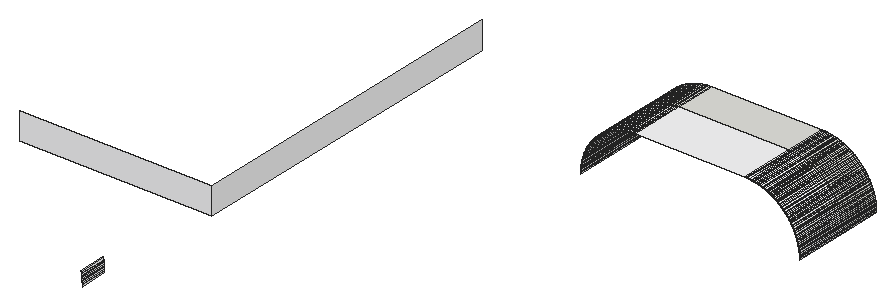
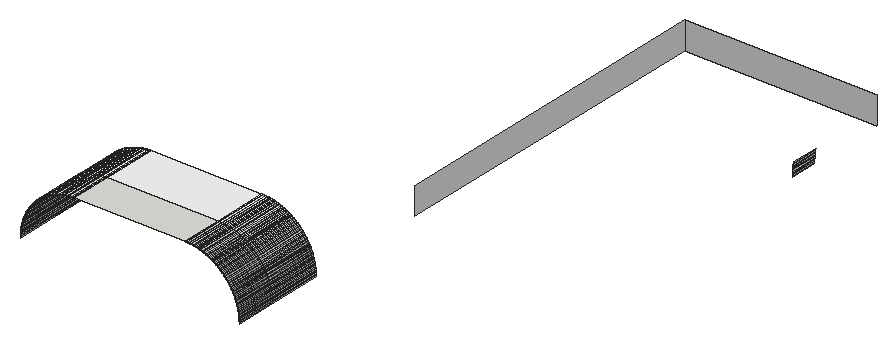
# SketchUp Ruby script. Lengths in inches.
U = 1.inch
M = Sketchup.active_model
def pt(a) = Geom::Point3d.new(a.map { |v| v * U })
def face(e, loops, mat)
  f = e.add_face(loops[0].map { |a| pt(a) })
  loops[1..].each { |l| e.add_face(l.map { |a| pt(a) }).erase! }
  f.material = f.back_material = mat if mat
  f
end
# faces: each face lists its corners as indices into pts; further lists are holes
def faces(e, pts, list, mat = nil) = list.each { |f| face(e, (f[0].is_a?(Array) ? f : [f]).map { |l| l.map { |i| pts[i] } }, mat) }
# xy, xz, yz: faces in a plane at the given z, y or x. An outline is a flat list of corners, or four numbers for a rectangle; further outlines are holes
def ring(l) = l.size == 4 ? [[l[0], l[1]], [l[2], l[1]], [l[2], l[3]], [l[0], l[3]]] : l.each_slice(2).to_a
def flat(e, list, mat, &to3) = list.each { |f| face(e, (f[0].is_a?(Array) ? f : [f]).map { |l| ring(l).map { |u, v| to3.(u, v) } }, mat) }
def xy(e, z, list, mat = nil) = flat(e, list, mat) { |x, y| [x, y, z] }
def xz(e, y, list, mat = nil) = flat(e, list, mat) { |x, z| [x, y, z] }
def yz(e, x, list, mat = nil) = flat(e, list, mat) { |y, z| [x, y, z] }
def lines(e, pts, list) = list.each { |a, b| e.add_line(pt(pts[a]), pt(pts[b])) }
# prism: a flat outline (further loops are holes) pulled along v
def prism(e, loops, v, mat = nil)
  f = face(e, loops, mat); d = Geom::Vector3d.new(v.map { |x| x * U })
  f.pushpull(f.normal.samedirection?(d) ? d.length : -d.length)
end
def box(e, o, s, mat = nil) = prism(e, [[o, [o[0] + s[0], o[1], o[2]], [o[0] + s[0], o[1] + s[1], o[2]], [o[0], o[1] + s[1], o[2]]]], [0, 0, s[2]], mat)
def at(x, y, z, deg = 0) = Geom::Transformation.translation(pt([x, y, z])) * Geom::Transformation.rotation(ORIGIN, Z_AXIS, deg.degrees)
def axes(o, x, y, z) = Geom::Transformation.new([*x, 0, *y, 0, *z, 0, *pt(o).to_a, 1])
def part(name) = M.definitions.add(name)
# library, detail: a bought-in or finely detailed component or shape, given as its bounding box
def library(name, o, s) = part(name).tap { |d| box(d.entities, o, s) }
def detail(e, o, s) = box(e.add_group.entities, o, s)
def put(e, d, t, mat = nil) = e.add_instance(d, t).tap { |i| i.material = mat if mat }
def group(e, t, mat = nil) = e.add_group.tap { |g| g.transformation = t; g.material = mat if mat }.entities
root = M.entities
M.materials.add("[Quartz Light Grey]").color = [251, 251, 252]
xy(root,222,[[245.6875,283,245.84,292],[245.84,283,246,292],[246,283,270,292],[270,283,270.16,292],[270.16,283,270.3125,292]])
xy(root,222,[[245.6875,271,245.84,283],[245.84,271,246,283],[246,271,270,283],[270,271,270.16,283],[270.16,271,270.3125,283]],"[Quartz Light Grey]")
xz(root,195,[[172,228,214,234]],"[Quartz Light Grey]")
yz(root,191.99,[[187,210.47,193,210.71]],"[Quartz Light Grey]")
yz(root,192,[[187,210,193,210.24]],"[Quartz Light Grey]")
yz(root,214,[[195,228,269,234]],"[Quartz Light Grey]")
yz(root,234,[[283,210,292,210.16],[283,210.16,292,210.3125]])
yz(root,234,[[271,210,283,210.16],[271,210.16,283,210.3125]],"[Quartz Light Grey]")
yz(root,282,[[283,210,292,210.16],[283,210.16,292,210.3125]])
yz(root,282,[[271,210,283,210.16],[271,210.16,283,210.3125]],"[Quartz Light Grey]")
p = [[191.99,187,210.47],[191.99,193,210.47],[192,193,210.24],[192,187,210.24],[234,283,210.3125],[234.01,283,210.47],
  [234.01,271,210.47],[234,271,210.3125],[281.99,283,210.47],[282,283,210.3125],[282,271,210.3125],[281.99,271,210.47],
  [234.01,292,210.47],[234.01,283,210.47],[234,283,210.3125],[234,292,210.3125],[282,292,210.3125],[282,283,210.3125],
  [281.99,283,210.47],[281.99,292,210.47],[234.02,283,210.63],[234.02,271,210.63],[281.98,283,210.63],[281.98,271,210.63],
  [234.02,292,210.63],[234.02,283,210.63],[281.98,283,210.63],[281.98,292,210.63],[234.03,283,210.78],[234.03,271,210.78],
  [281.97,283,210.78],[281.97,271,210.78],[234.03,292,210.78],[234.03,283,210.78],[281.97,283,210.78],[281.97,292,210.78],
  [191.98,187,210.94],[191.98,193,210.94],[191.99,193,210.71],[191.99,187,210.71],[234.04,283,210.94],[234.04,271,210.94],
  [281.96,283,210.94],[281.96,271,210.94],[234.04,292,210.94],[234.04,283,210.94],[281.96,283,210.94],[281.96,292,210.94],
  [191.96,187,211.18],[191.96,193,211.18],[234.05,283,211.1],[234.05,271,211.1],[281.95,283,211.1],[281.95,271,211.1],
  [234.05,292,211.1],[234.05,283,211.1],[281.95,283,211.1],[281.95,292,211.1],[234.07,283,211.25],[234.07,271,211.25],
  [281.93,283,211.25],[281.93,271,211.25],[234.07,292,211.25],[234.07,283,211.25],[281.93,283,211.25],[281.93,292,211.25],
  [191.94,187,211.41],[191.94,193,211.41],[234.08,283,211.41],[234.08,271,211.41],[281.92,283,211.41],[281.92,271,211.41],
  [234.08,292,211.41],[234.08,283,211.41],[281.92,283,211.41],[281.92,292,211.41],[191.92,187,211.65],[191.92,193,211.65],
  [234.1,283,211.57],[234.1,271,211.57],[281.9,283,211.57],[281.9,271,211.57],[234.1,292,211.57],[234.1,283,211.57],
  [281.9,283,211.57],[281.9,292,211.57],[191.9,187,211.88],[191.9,193,211.88],[234.125,283,211.72],[234.125,271,211.72],
  [281.875,283,211.72],[281.875,271,211.72],[234.125,292,211.72],[234.125,283,211.72],[281.875,283,211.72],[281.875,292,211.72],
  [234.15,283,211.88],[234.15,271,211.88],[281.85,283,211.88],[281.85,271,211.88],[234.15,292,211.88],[234.15,283,211.88],
  [281.85,283,211.88],[281.85,292,211.88],[191.875,187,212.12],[191.875,193,212.12],[234.17,283,212.03],[234.17,271,212.03],
  [281.83,283,212.03],[281.83,271,212.03],[234.17,292,212.03],[234.17,283,212.03],[281.83,283,212.03],[281.83,292,212.03],
  [234.2,283,212.1875],[234.2,271,212.1875],[281.8,283,212.1875],[281.8,271,212.1875],[234.2,292,212.1875],[234.2,283,212.1875],
  [281.8,283,212.1875],[281.8,292,212.1875],[191.85,187,212.35],[191.85,193,212.35],[234.23,283,212.34],[234.23,271,212.34],
  [281.77,283,212.34],[281.77,271,212.34],[234.23,292,212.34],[234.23,283,212.34],[281.77,283,212.34],[281.77,292,212.34],
  [191.8125,187,212.58],[191.8125,193,212.58],[234.26,283,212.49],[234.26,271,212.49],[281.74,283,212.49],[281.74,271,212.49],
  [234.26,292,212.49],[234.26,283,212.49],[281.74,283,212.49],[281.74,292,212.49],[234.3,283,212.65],[234.3,271,212.65],
  [281.7,283,212.65],[281.7,271,212.65],[234.3,292,212.65],[234.3,283,212.65],[281.7,283,212.65],[281.7,292,212.65],
  [191.78,187,212.82],[191.78,193,212.82],[234.33,283,212.8],[234.33,271,212.8],[281.67,283,212.8],[281.67,271,212.8],
  [234.33,292,212.8],[234.33,283,212.8],[281.67,283,212.8],[281.67,292,212.8],[191.74,187,213.05],[191.74,193,213.05],
  [234.37,283,212.95],[234.37,271,212.95],[281.63,283,212.95],[281.63,271,212.95],[234.37,292,212.95],[234.37,283,212.95],
  [281.63,283,212.95],[281.63,292,212.95],[234.41,283,213.11],[234.41,271,213.11],[281.59,283,213.11],[281.59,271,213.11],
  [234.41,292,213.11],[234.41,283,213.11],[281.59,283,213.11],[281.59,292,213.11],[234.45,283,213.26],[234.45,271,213.26],
  [281.55,283,213.26],[281.55,271,213.26],[234.45,292,213.26],[234.45,283,213.26],[281.55,283,213.26],[281.55,292,213.26],
  [234.49,283,213.41],[234.49,271,213.41],[281.51,283,213.41],[281.51,271,213.41],[234.49,292,213.41],[234.49,283,213.41],
  [281.51,283,213.41],[281.51,292,213.41],[234.54,283,213.56],[234.54,271,213.56],[281.46,283,213.56],[281.46,271,213.56],
  [234.54,292,213.56],[234.54,283,213.56],[281.46,283,213.56],[281.46,292,213.56],[234.59,283,213.71],[234.59,271,213.71],
  [281.41,283,213.71],[281.41,271,213.71],[234.59,292,213.71],[234.59,283,213.71],[281.41,283,213.71],[281.41,292,213.71],
  [234.64,283,213.86],[234.64,271,213.86],[281.36,283,213.86],[281.36,271,213.86],[234.64,292,213.86],[234.64,283,213.86],
  [281.36,283,213.86],[281.36,292,213.86],[234.6875,283,214.01],[234.6875,271,214.01],[281.3125,283,214.01],[281.3125,271,214.01],
  [234.6875,292,214.01],[234.6875,283,214.01],[281.3125,283,214.01],[281.3125,292,214.01],[234.74,283,214.15],[234.74,271,214.15],
  [281.26,283,214.15],[281.26,271,214.15],[234.74,292,214.15],[234.74,283,214.15],[281.26,283,214.15],[281.26,292,214.15],
  [234.8,283,214.3],[234.8,271,214.3],[281.2,283,214.3],[281.2,271,214.3],[234.8,292,214.3],[234.8,283,214.3],
  [281.2,283,214.3],[281.2,292,214.3],[234.85,283,214.45],[234.85,271,214.45],[281.15,283,214.45],[281.15,271,214.45],
  [234.85,292,214.45],[234.85,283,214.45],[281.15,283,214.45],[281.15,292,214.45],[234.91,283,214.59],[234.91,271,214.59],
  [281.09,283,214.59],[281.09,271,214.59],[234.91,292,214.59],[234.91,283,214.59],[281.09,283,214.59],[281.09,292,214.59],
  [234.97,283,214.74],[234.97,271,214.74],[281.03,283,214.74],[281.03,271,214.74],[234.97,292,214.74],[234.97,283,214.74],
  [281.03,283,214.74],[281.03,292,214.74],[235.04,283,214.88],[235.04,271,214.88],[280.96,283,214.88],[280.96,271,214.88],
  [235.04,292,214.88],[235.04,283,214.88],[280.96,283,214.88],[280.96,292,214.88],[235.1,283,215.02],[235.1,271,215.02],
  [280.9,283,215.02],[280.9,271,215.02],[235.1,292,215.02],[235.1,283,215.02],[280.9,283,215.02],[280.9,292,215.02],
  [235.17,283,215.17],[235.17,271,215.17],[280.83,283,215.17],[280.83,271,215.17],[235.17,292,215.17],[235.17,283,215.17],
  [280.83,283,215.17],[280.83,292,215.17],[235.24,283,215.31],[235.24,271,215.31],[280.76,283,215.31],[280.76,271,215.31],
  [235.24,292,215.31],[235.24,283,215.31],[280.76,283,215.31],[280.76,292,215.31],[235.31,283,215.45],[235.31,271,215.45],
  [280.69,283,215.45],[280.69,271,215.45],[235.31,292,215.45],[235.31,283,215.45],[280.69,283,215.45],[280.69,292,215.45],
  [235.38,283,215.59],[235.38,271,215.59],[280.62,283,215.59],[280.62,271,215.59],[235.38,292,215.59],[235.38,283,215.59],
  [280.62,283,215.59],[280.62,292,215.59],[235.45,283,215.73],[235.45,271,215.73],[280.55,283,215.73],[280.55,271,215.73],
  [235.45,292,215.73],[235.45,283,215.73],[280.55,283,215.73],[280.55,292,215.73],[235.53,283,215.86],[235.53,271,215.86],
  [280.47,283,215.86],[280.47,271,215.86],[235.53,292,215.86],[235.53,283,215.86],[280.47,283,215.86],[280.47,292,215.86],
  [235.61,283,216],[235.61,271,216],[280.39,283,216],[280.39,271,216],[235.61,292,216],[235.61,283,216],
  [280.39,283,216],[280.39,292,216],[235.6875,283,216.14],[235.6875,271,216.14],[280.3125,283,216.14],[280.3125,271,216.14],
  [235.6875,292,216.14],[235.6875,283,216.14],[280.3125,283,216.14],[280.3125,292,216.14],[235.77,283,216.27],[235.77,271,216.27],
  [280.23,283,216.27],[280.23,271,216.27],[235.77,292,216.27],[235.77,283,216.27],[280.23,283,216.27],[280.23,292,216.27],
  [235.85,283,216.4],[235.85,271,216.4],[280.15,283,216.4],[280.15,271,216.4],[235.85,292,216.4],[235.85,283,216.4],
  [280.15,283,216.4],[280.15,292,216.4],[235.9375,283,216.54],[235.9375,271,216.54],[280.0625,283,216.54],[280.0625,271,216.54],
  [235.9375,292,216.54],[235.9375,283,216.54],[280.0625,283,216.54],[280.0625,292,216.54],[236.02,283,216.67],[236.02,271,216.67],
  [279.98,283,216.67],[279.98,271,216.67],[236.02,292,216.67],[236.02,283,216.67],[279.98,283,216.67],[279.98,292,216.67],
  [236.11,283,216.8],[236.11,271,216.8],[279.89,283,216.8],[279.89,271,216.8],[236.11,292,216.8],[236.11,283,216.8],
  [279.89,283,216.8],[279.89,292,216.8],[236.2,283,216.93],[236.2,271,216.93],[279.8,283,216.93],[279.8,271,216.93],
  [236.2,292,216.93],[236.2,283,216.93],[279.8,283,216.93],[279.8,292,216.93],[236.29,283,217.05],[236.29,271,217.05],
  [279.71,283,217.05],[279.71,271,217.05],[236.29,292,217.05],[236.29,283,217.05],[279.71,283,217.05],[279.71,292,217.05],
  [236.38,283,217.18],[236.38,271,217.18],[279.62,283,217.18],[279.62,271,217.18],[236.38,292,217.18],[236.38,283,217.18],
  [279.62,283,217.18],[279.62,292,217.18],[236.48,283,217.31],[236.48,271,217.31],[279.52,283,217.31],[279.52,271,217.31],
  [236.48,292,217.31],[236.48,283,217.31],[279.52,283,217.31],[279.52,292,217.31],[236.58,283,217.43],[236.58,271,217.43],
  [279.42,283,217.43],[279.42,271,217.43],[236.58,292,217.43],[236.58,283,217.43],[279.42,283,217.43],[279.42,292,217.43],
  [236.67,283,217.55],[236.67,271,217.55],[279.33,283,217.55],[279.33,271,217.55],[236.67,292,217.55],[236.67,283,217.55],
  [279.33,283,217.55],[279.33,292,217.55],[236.77,283,217.67],[236.77,271,217.67],[279.23,283,217.67],[279.23,271,217.67],
  [236.77,292,217.67],[236.77,283,217.67],[279.23,283,217.67],[279.23,292,217.67],[236.875,283,217.79],[236.875,271,217.79],
  [279.125,283,217.79],[279.125,271,217.79],[236.875,292,217.79],[236.875,283,217.79],[279.125,283,217.79],[279.125,292,217.79],
  [236.98,283,217.91],[236.98,271,217.91],[279.02,283,217.91],[279.02,271,217.91],[236.98,292,217.91],[236.98,283,217.91],
  [279.02,283,217.91],[279.02,292,217.91],[237.08,283,218.03],[237.08,271,218.03],[278.92,283,218.03],[278.92,271,218.03],
  [237.08,292,218.03],[237.08,283,218.03],[278.92,283,218.03],[278.92,292,218.03],[237.1875,283,218.15],[237.1875,271,218.15],
  [278.8125,283,218.15],[278.8125,271,218.15],[237.1875,292,218.15],[237.1875,283,218.15],[278.8125,283,218.15],[278.8125,292,218.15],
  [237.3,283,218.26],[237.3,271,218.26],[278.7,283,218.26],[278.7,271,218.26],[237.3,292,218.26],[237.3,283,218.26],
  [278.7,283,218.26],[278.7,292,218.26],[237.4,283,218.375],[237.4,271,218.375],[278.6,283,218.375],[278.6,271,218.375],
  [237.4,292,218.375],[237.4,283,218.375],[278.6,283,218.375],[278.6,292,218.375],[237.51,283,218.49],[237.51,271,218.49],
  [278.49,283,218.49],[278.49,271,218.49],[237.51,292,218.49],[237.51,283,218.49],[278.49,283,218.49],[278.49,292,218.49],
  [237.625,283,218.6],[237.625,271,218.6],[278.375,283,218.6],[278.375,271,218.6],[237.625,292,218.6],[237.625,283,218.6],
  [278.375,283,218.6],[278.375,292,218.6],[237.74,283,218.7],[237.74,271,218.7],[278.26,283,218.7],[278.26,271,218.7],
  [237.74,292,218.7],[237.74,283,218.7],[278.26,283,218.7],[278.26,292,218.7],[237.85,283,218.8125],[237.85,271,218.8125],
  [278.15,283,218.8125],[278.15,271,218.8125],[237.85,292,218.8125],[237.85,283,218.8125],[278.15,283,218.8125],[278.15,292,218.8125],
  [237.97,283,218.92],[237.97,271,218.92],[278.03,283,218.92],[278.03,271,218.92],[237.97,292,218.92],[237.97,283,218.92],
  [278.03,283,218.92],[278.03,292,218.92],[238.09,283,219.02],[238.09,271,219.02],[277.91,283,219.02],[277.91,271,219.02],
  [238.09,292,219.02],[238.09,283,219.02],[277.91,283,219.02],[277.91,292,219.02],[238.21,283,219.125],[238.21,271,219.125],
  [277.79,283,219.125],[277.79,271,219.125],[238.21,292,219.125],[238.21,283,219.125],[277.79,283,219.125],[277.79,292,219.125],
  [238.33,283,219.23],[238.33,271,219.23],[277.67,283,219.23],[277.67,271,219.23],[238.33,292,219.23],[238.33,283,219.23],
  [277.67,283,219.23],[277.67,292,219.23],[238.45,283,219.33],[238.45,271,219.33],[277.55,283,219.33],[277.55,271,219.33],
  [238.45,292,219.33],[238.45,283,219.33],[277.55,283,219.33],[277.55,292,219.33],[238.57,283,219.42],[238.57,271,219.42],
  [277.43,283,219.42],[277.43,271,219.42],[238.57,292,219.42],[238.57,283,219.42],[277.43,283,219.42],[277.43,292,219.42],
  [238.69,283,219.52],[238.69,271,219.52],[277.31,283,219.52],[277.31,271,219.52],[238.69,292,219.52],[238.69,283,219.52],
  [277.31,283,219.52],[277.31,292,219.52],[238.82,283,219.62],[238.82,271,219.62],[277.18,283,219.62],[277.18,271,219.62],
  [238.82,292,219.62],[238.82,283,219.62],[277.18,283,219.62],[277.18,292,219.62],[238.95,283,219.71],[238.95,271,219.71],
  [277.05,283,219.71],[277.05,271,219.71],[238.95,292,219.71],[238.95,283,219.71],[277.05,283,219.71],[277.05,292,219.71],
  [239.07,283,219.8],[239.07,271,219.8],[276.93,283,219.8],[276.93,271,219.8],[239.07,292,219.8],[239.07,283,219.8],
  [276.93,283,219.8],[276.93,292,219.8],[239.2,283,219.89],[239.2,271,219.89],[276.8,283,219.89],[276.8,271,219.89],
  [239.2,292,219.89],[239.2,283,219.89],[276.8,283,219.89],[276.8,292,219.89],[239.33,283,219.98],[239.33,271,219.98],
  [276.67,283,219.98],[276.67,271,219.98],[239.33,292,219.98],[239.33,283,219.98],[276.67,283,219.98],[276.67,292,219.98],
  [239.46,283,220.0625],[239.46,271,220.0625],[276.54,283,220.0625],[276.54,271,220.0625],[239.46,292,220.0625],[239.46,283,220.0625],
  [276.54,283,220.0625],[276.54,292,220.0625],[239.6,283,220.15],[239.6,271,220.15],[239.73,283,220.23],[239.73,271,220.23],
  [276.27,283,220.23],[276.4,283,220.15],[276.4,271,220.15],[276.27,271,220.23],[239.6,292,220.15],[239.6,283,220.15],
  [239.73,292,220.23],[239.73,283,220.23],[276.4,292,220.15],[276.4,283,220.15],[276.27,283,220.23],[276.27,292,220.23],
  [239.86,283,220.3125],[239.86,271,220.3125],[276.14,283,220.3125],[276.14,271,220.3125],[239.86,292,220.3125],[239.86,283,220.3125],
  [276.14,283,220.3125],[276.14,292,220.3125],[240,283,220.39],[240,271,220.39],[276,283,220.39],[276,271,220.39],
  [240,292,220.39],[240,283,220.39],[276,283,220.39],[276,292,220.39],[240.14,283,220.47],[240.14,271,220.47],
  [275.86,283,220.47],[275.86,271,220.47],[240.14,292,220.47],[240.14,283,220.47],[275.86,283,220.47],[275.86,292,220.47],
  [240.27,283,220.55],[240.27,271,220.55],[240.41,283,220.62],[240.41,271,220.62],[275.59,283,220.62],[275.73,283,220.55],
  [275.73,271,220.55],[275.59,271,220.62],[240.27,292,220.55],[240.27,283,220.55],[240.41,292,220.62],[240.41,283,220.62],
  [275.73,292,220.55],[275.73,283,220.55],[275.59,283,220.62],[275.59,292,220.62],[240.55,283,220.69],[240.55,271,220.69],
  [275.45,283,220.69],[275.45,271,220.69],[240.55,292,220.69],[240.55,283,220.69],[275.45,283,220.69],[275.45,292,220.69],
  [240.69,283,220.76],[240.69,271,220.76],[275.31,283,220.76],[275.31,271,220.76],[240.69,292,220.76],[240.69,283,220.76],
  [275.31,283,220.76],[275.31,292,220.76],[240.83,283,220.83],[240.83,271,220.83],[240.98,283,220.9],[240.98,271,220.9],
  [275.02,283,220.9],[275.17,283,220.83],[275.17,271,220.83],[275.02,271,220.9],[240.83,292,220.83],[240.83,283,220.83],
  [240.98,292,220.9],[240.98,283,220.9],[275.17,292,220.83],[275.17,283,220.83],[275.02,283,220.9],[275.02,292,220.9],
  [241.12,283,220.96],[241.12,271,220.96],[274.88,283,220.96],[274.88,271,220.96],[241.12,292,220.96],[241.12,283,220.96],
  [274.88,283,220.96],[274.88,292,220.96],[241.26,283,221.03],[241.26,271,221.03],[241.41,283,221.09],[241.41,271,221.09],
  [274.59,283,221.09],[274.74,283,221.03],[274.74,271,221.03],[274.59,271,221.09],[241.26,292,221.03],[241.26,283,221.03],
  [241.41,292,221.09],[241.41,283,221.09],[274.74,292,221.03],[274.74,283,221.03],[274.59,283,221.09],[274.59,292,221.09],
  [241.55,283,221.15],[241.55,271,221.15],[241.7,283,221.2],[241.7,271,221.2],[274.3,283,221.2],[274.45,283,221.15],
  [274.45,271,221.15],[274.3,271,221.2],[241.55,292,221.15],[241.55,283,221.15],[241.7,292,221.2],[241.7,283,221.2],
  [274.45,292,221.15],[274.45,283,221.15],[274.3,283,221.2],[274.3,292,221.2],[241.85,283,221.26],[241.85,271,221.26],
  [274.15,283,221.26],[274.15,271,221.26],[241.85,292,221.26],[241.85,283,221.26],[274.15,283,221.26],[274.15,292,221.26],
  [241.99,283,221.3125],[241.99,271,221.3125],[242.14,283,221.36],[242.14,271,221.36],[273.86,283,221.36],[274.01,283,221.3125],
  [274.01,271,221.3125],[273.86,271,221.36],[241.99,292,221.3125],[241.99,283,221.3125],[242.14,292,221.36],[242.14,283,221.36],
  [274.01,292,221.3125],[274.01,283,221.3125],[273.86,283,221.36],[273.86,292,221.36],[242.29,283,221.41],[242.29,271,221.41],
  [242.44,283,221.46],[242.44,271,221.46],[273.56,283,221.46],[273.71,283,221.41],[273.71,271,221.41],[273.56,271,221.46],
  [242.29,292,221.41],[242.29,283,221.41],[242.44,292,221.46],[242.44,283,221.46],[273.71,292,221.41],[273.71,283,221.41],
  [273.56,283,221.46],[273.56,292,221.46],[242.59,283,221.51],[242.59,271,221.51],[242.74,283,221.55],[242.74,271,221.55],
  [242.89,283,221.59],[242.89,271,221.59],[273.11,283,221.59],[273.26,283,221.55],[273.26,271,221.55],[273.11,271,221.59],
  [273.41,283,221.51],[273.41,271,221.51],[242.59,292,221.51],[242.59,283,221.51],[242.74,292,221.55],[242.74,283,221.55],
  [242.89,292,221.59],[242.89,283,221.59],[273.26,292,221.55],[273.26,283,221.55],[273.11,283,221.59],[273.11,292,221.59],
  [273.41,292,221.51],[273.41,283,221.51],[243.05,283,221.63],[243.05,271,221.63],[243.2,283,221.67],[243.2,271,221.67],
  [272.8,283,221.67],[272.95,283,221.63],[272.95,271,221.63],[272.8,271,221.67],[243.05,292,221.63],[243.05,283,221.63],
  [243.2,292,221.67],[243.2,283,221.67],[272.95,292,221.63],[272.95,283,221.63],[272.8,283,221.67],[272.8,292,221.67],
  [243.35,283,221.7],[243.35,271,221.7],[243.51,283,221.74],[243.51,271,221.74],[243.66,283,221.77],[243.66,271,221.77],
  [272.34,283,221.77],[272.49,283,221.74],[272.49,271,221.74],[272.34,271,221.77],[272.65,283,221.7],[272.65,271,221.7],
  [243.35,292,221.7],[243.35,283,221.7],[243.51,292,221.74],[243.51,283,221.74],[243.66,292,221.77],[243.66,283,221.77],
  [272.49,292,221.74],[272.49,283,221.74],[272.34,283,221.77],[272.34,292,221.77],[272.65,292,221.7],[272.65,283,221.7],
  [243.8125,283,221.8],[243.8125,271,221.8],[243.97,283,221.83],[243.97,271,221.83],[244.12,283,221.85],[244.12,271,221.85],
  [271.88,283,221.85],[272.03,283,221.83],[272.03,271,221.83],[271.88,271,221.85],[272.1875,283,221.8],[272.1875,271,221.8],
  [243.8125,292,221.8],[243.8125,283,221.8],[243.97,292,221.83],[243.97,283,221.83],[244.12,292,221.85],[244.12,283,221.85],
  [272.03,292,221.83],[272.03,283,221.83],[271.88,283,221.85],[271.88,292,221.85],[272.1875,292,221.8],[272.1875,283,221.8],
  [244.28,283,221.875],[244.28,271,221.875],[244.43,283,221.9],[244.43,271,221.9],[244.59,283,221.92],[244.59,271,221.92],
  [244.75,283,221.93],[244.75,271,221.93],[244.9,283,221.95],[244.9,271,221.95],[245.06,283,221.96],[245.06,271,221.96],
  [270.94,283,221.96],[271.1,283,221.95],[271.1,271,221.95],[270.94,271,221.96],[271.25,283,221.93],[271.25,271,221.93],
  [271.41,283,221.92],[271.41,271,221.92],[271.57,283,221.9],[271.57,271,221.9],[271.72,283,221.875],[271.72,271,221.875],
  [244.28,292,221.875],[244.28,283,221.875],[244.43,292,221.9],[244.43,283,221.9],[244.59,292,221.92],[244.59,283,221.92],
  [244.75,292,221.93],[244.75,283,221.93],[244.9,292,221.95],[244.9,283,221.95],[245.06,292,221.96],[245.06,283,221.96],
  [271.1,292,221.95],[271.1,283,221.95],[270.94,283,221.96],[270.94,292,221.96],[271.25,292,221.93],[271.25,283,221.93],
  [271.41,292,221.92],[271.41,283,221.92],[271.57,292,221.9],[271.57,283,221.9],[271.72,292,221.875],[271.72,283,221.875],
  [245.22,283,221.97],[245.22,271,221.97],[245.37,283,221.98],[245.37,271,221.98],[245.53,283,221.99],[245.53,271,221.99],
  [245.6875,283,222],[245.6875,271,222],[270.3125,283,222],[270.47,283,221.99],[270.47,271,221.99],[270.3125,271,222],
  [270.63,283,221.98],[270.63,271,221.98],[270.78,283,221.97],[270.78,271,221.97],[245.22,292,221.97],[245.22,283,221.97],
  [245.37,292,221.98],[245.37,283,221.98],[245.53,292,221.99],[245.53,283,221.99],[245.6875,292,222],[245.6875,283,222],
  [270.47,292,221.99],[270.47,283,221.99],[270.3125,283,222],[270.3125,292,222],[270.63,292,221.98],[270.63,283,221.98],
  [270.78,292,221.97],[270.78,283,221.97]]
faces(root,p,[[0,1,2,3],[4,5,6,7],[8,9,10,11],[5,20,21,6],[22,8,11,23],[20,28,29,21],[30,22,23,31],[36,37,38,39],
  [28,40,41,29],[42,30,31,43],[48,49,37,36],[40,50,51,41],[52,42,43,53],[50,58,59,51],[60,52,53,61],[66,67,49,48],
  [58,68,69,59],[70,60,61,71],[76,77,67,66],[68,78,79,69],[80,70,71,81],[86,87,77,76],[78,88,89,79],[90,80,81,91],
  [88,96,97,89],[98,90,91,99],[104,105,87,86],[96,106,107,97],[108,98,99,109],[106,114,115,107],[116,108,109,117],[122,123,105,104],
  [114,124,125,115],[126,116,117,127],[132,133,123,122],[124,134,135,125],[136,126,127,137],[134,142,143,135],[144,136,137,145],[150,151,133,132],
  [142,152,153,143],[154,144,145,155],[160,161,151,150],[152,162,163,153],[164,154,155,165],[162,170,171,163],[172,164,165,173],[170,178,179,171],
  [180,172,173,181],[178,186,187,179],[188,180,181,189],[186,194,195,187],[196,188,189,197],[194,202,203,195],[204,196,197,205],[202,210,211,203],
  [212,204,205,213],[210,218,219,211],[220,212,213,221],[218,226,227,219],[228,220,221,229],[226,234,235,227],[236,228,229,237],[234,242,243,235],
  [244,236,237,245],[242,250,251,243],[252,244,245,253],[250,258,259,251],[260,252,253,261],[258,266,267,259],[268,260,261,269],[266,274,275,267],
  [276,268,269,277],[274,282,283,275],[284,276,277,285],[282,290,291,283],[292,284,285,293],[290,298,299,291],[300,292,293,301],[298,306,307,299],
  [308,300,301,309],[306,314,315,307],[316,308,309,317],[314,322,323,315],[324,316,317,325],[322,330,331,323],[332,324,325,333],[330,338,339,331],
  [340,332,333,341],[338,346,347,339],[348,340,341,349],[346,354,355,347],[356,348,349,357],[354,362,363,355],[364,356,357,365],[362,370,371,363],
  [372,364,365,373],[370,378,379,371],[380,372,373,381],[378,386,387,379],[388,380,381,389],[386,394,395,387],[396,388,389,397],[394,402,403,395],
  [404,396,397,405],[402,410,411,403],[412,404,405,413],[410,418,419,411],[420,412,413,421],[418,426,427,419],[428,420,421,429],[426,434,435,427],
  [436,428,429,437],[434,442,443,435],[444,436,437,445],[442,450,451,443],[452,444,445,453],[450,458,459,451],[460,452,453,461],[458,466,467,459],
  [468,460,461,469],[466,474,475,467],[476,468,469,477],[474,482,483,475],[484,476,477,485],[482,490,491,483],[492,484,485,493],[490,498,499,491],
  [500,492,493,501],[498,506,507,499],[508,500,501,509],[506,514,515,507],[516,508,509,517],[514,522,523,515],[524,516,517,525],[522,530,531,523],
  [532,524,525,533],[530,538,539,531],[540,532,533,541],[538,546,547,539],[548,540,541,549],[546,554,555,547],[556,548,549,557],[554,562,563,555],
  [564,556,557,565],[562,570,571,563],[572,564,565,573],[570,578,579,571],[580,572,573,581],[578,586,587,579],[588,580,581,589],[586,594,595,587],
  [596,588,589,597],[594,602,603,595],[604,596,597,605],[602,610,611,603],[612,604,605,613],[610,618,619,611],[620,612,613,621],[618,626,627,619],
  [626,628,629,627],[630,631,632,633],[631,620,621,632],[628,642,643,629],[644,630,633,645],[642,650,651,643],[652,644,645,653],[650,658,659,651],
  [660,652,653,661],[658,666,667,659],[666,668,669,667],[670,671,672,673],[671,660,661,672],[668,682,683,669],[684,670,673,685],[682,690,691,683],
  [692,684,685,693],[690,698,699,691],[698,700,701,699],[702,703,704,705],[703,692,693,704],[700,714,715,701],[716,702,705,717],[714,722,723,715],
  [722,724,725,723],[726,727,728,729],[727,716,717,728],[724,738,739,725],[738,740,741,739],[742,743,744,745],[743,726,729,744],[740,754,755,741],
  [756,742,745,757],[754,762,763,755],[762,764,765,763],[766,767,768,769],[767,756,757,768],[764,778,779,765],[778,780,781,779],[782,783,784,785],
  [783,766,769,784],[780,794,795,781],[794,796,797,795],[796,798,799,797],[800,801,802,803],[801,804,805,802],[804,782,785,805],[798,818,819,799],
  [818,820,821,819],[822,823,824,825],[823,800,803,824],[820,834,835,821],[834,836,837,835],[836,838,839,837],[840,841,842,843],[841,844,845,842],
  [844,822,825,845],[838,858,859,839],[858,860,861,859],[860,862,863,861],[864,865,866,867],[865,868,869,866],[868,840,843,869],[862,882,883,863],
  [882,884,885,883],[884,886,887,885],[886,888,889,887],[888,890,891,889],[890,892,893,891],[894,895,896,897],[895,898,899,896],[898,900,901,899],
  [900,902,903,901],[902,904,905,903],[904,864,867,905],[892,930,931,893],[930,932,933,931],[932,934,935,933],[934,936,937,935],[938,939,940,941],
  [939,942,943,940],[942,944,945,943],[944,894,897,945]],"[Quartz Light Grey]")
faces(root,p,[[12,13,14,15],[16,17,18,19],[24,25,13,12],[19,18,26,27],[32,33,25,24],[27,26,34,35],[44,45,33,32],[35,34,46,47],
  [54,55,45,44],[47,46,56,57],[62,63,55,54],[57,56,64,65],[72,73,63,62],[65,64,74,75],[82,83,73,72],[75,74,84,85],
  [92,93,83,82],[85,84,94,95],[100,101,93,92],[95,94,102,103],[110,111,101,100],[103,102,112,113],[118,119,111,110],[113,112,120,121],
  [128,129,119,118],[121,120,130,131],[138,139,129,128],[131,130,140,141],[146,147,139,138],[141,140,148,149],[156,157,147,146],[149,148,158,159],
  [166,167,157,156],[159,158,168,169],[174,175,167,166],[169,168,176,177],[182,183,175,174],[177,176,184,185],[190,191,183,182],[185,184,192,193],
  [198,199,191,190],[193,192,200,201],[206,207,199,198],[201,200,208,209],[214,215,207,206],[209,208,216,217],[222,223,215,214],[217,216,224,225],
  [230,231,223,222],[225,224,232,233],[238,239,231,230],[233,232,240,241],[246,247,239,238],[241,240,248,249],[254,255,247,246],[249,248,256,257],
  [262,263,255,254],[257,256,264,265],[270,271,263,262],[265,264,272,273],[278,279,271,270],[273,272,280,281],[286,287,279,278],[281,280,288,289],
  [294,295,287,286],[289,288,296,297],[302,303,295,294],[297,296,304,305],[310,311,303,302],[305,304,312,313],[318,319,311,310],[313,312,320,321],
  [326,327,319,318],[321,320,328,329],[334,335,327,326],[329,328,336,337],[342,343,335,334],[337,336,344,345],[350,351,343,342],[345,344,352,353],
  [358,359,351,350],[353,352,360,361],[366,367,359,358],[361,360,368,369],[374,375,367,366],[369,368,376,377],[382,383,375,374],[377,376,384,385],
  [390,391,383,382],[385,384,392,393],[398,399,391,390],[393,392,400,401],[406,407,399,398],[401,400,408,409],[414,415,407,406],[409,408,416,417],
  [422,423,415,414],[417,416,424,425],[430,431,423,422],[425,424,432,433],[438,439,431,430],[433,432,440,441],[446,447,439,438],[441,440,448,449],
  [454,455,447,446],[449,448,456,457],[462,463,455,454],[457,456,464,465],[470,471,463,462],[465,464,472,473],[478,479,471,470],[473,472,480,481],
  [486,487,479,478],[481,480,488,489],[494,495,487,486],[489,488,496,497],[502,503,495,494],[497,496,504,505],[510,511,503,502],[505,504,512,513],
  [518,519,511,510],[513,512,520,521],[526,527,519,518],[521,520,528,529],[534,535,527,526],[529,528,536,537],[542,543,535,534],[537,536,544,545],
  [550,551,543,542],[545,544,552,553],[558,559,551,550],[553,552,560,561],[566,567,559,558],[561,560,568,569],[574,575,567,566],[569,568,576,577],
  [582,583,575,574],[577,576,584,585],[590,591,583,582],[585,584,592,593],[598,599,591,590],[593,592,600,601],[606,607,599,598],[601,600,608,609],
  [614,615,607,606],[609,608,616,617],[622,623,615,614],[617,616,624,625],[634,635,623,622],[636,637,635,634],[638,639,640,641],[625,624,639,638],
  [646,647,637,636],[641,640,648,649],[654,655,647,646],[649,648,656,657],[662,663,655,654],[657,656,664,665],[674,675,663,662],[676,677,675,674],
  [678,679,680,681],[665,664,679,678],[686,687,677,676],[681,680,688,689],[694,695,687,686],[689,688,696,697],[706,707,695,694],[708,709,707,706],
  [710,711,712,713],[697,696,711,710],[718,719,709,708],[713,712,720,721],[730,731,719,718],[732,733,731,730],[734,735,736,737],[721,720,735,734],
  [746,747,733,732],[748,749,747,746],[750,751,752,753],[737,736,751,750],[758,759,749,748],[753,752,760,761],[770,771,759,758],[772,773,771,770],
  [774,775,776,777],[761,760,775,774],[786,787,773,772],[788,789,787,786],[790,791,792,793],[777,776,791,790],[806,807,789,788],[808,809,807,806],
  [810,811,809,808],[812,813,814,815],[816,817,813,812],[793,792,817,816],[826,827,811,810],[828,829,827,826],[830,831,832,833],[815,814,831,830],
  [846,847,829,828],[848,849,847,846],[850,851,849,848],[852,853,854,855],[856,857,853,852],[833,832,857,856],[870,871,851,850],[872,873,871,870],
  [874,875,873,872],[876,877,878,879],[880,881,877,876],[855,854,881,880],[906,907,875,874],[908,909,907,906],[910,911,909,908],[912,913,911,910],
  [914,915,913,912],[916,917,915,914],[918,919,920,921],[922,923,919,918],[924,925,923,922],[926,927,925,924],[928,929,927,926],[879,878,929,928],
  [946,947,917,916],[948,949,947,946],[950,951,949,948],[952,953,951,950],[954,955,956,957],[958,959,955,954],[960,961,959,958],[921,920,961,960]])
